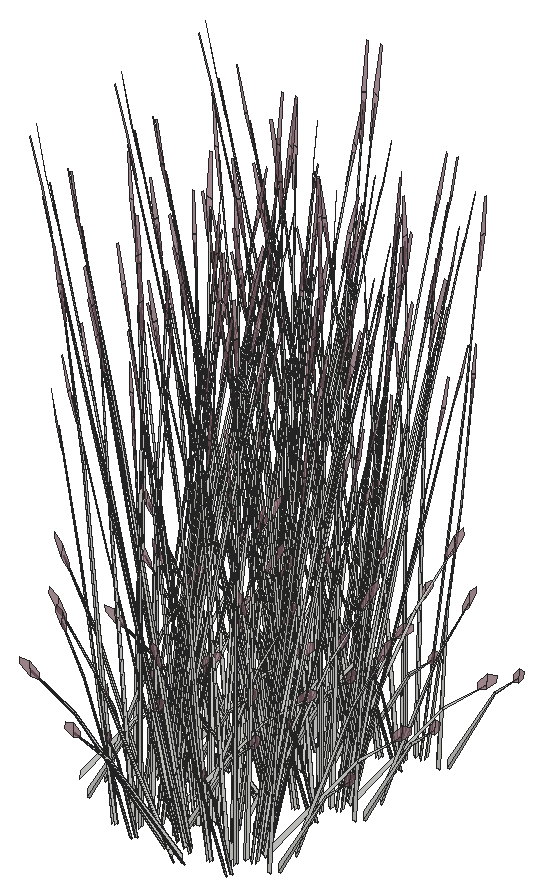
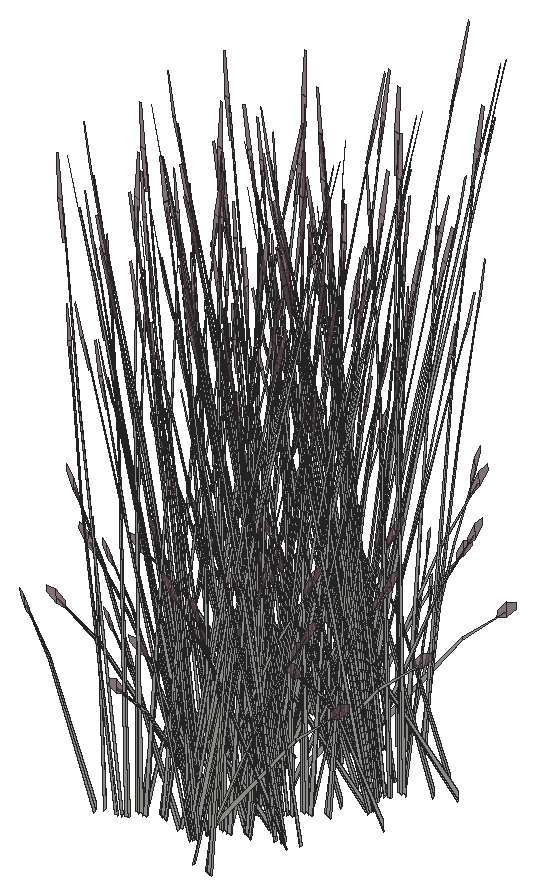
# SketchUp Ruby script. Lengths in inches.
U = 1.inch
M = Sketchup.active_model
def pt(a) = Geom::Point3d.new(a.map { |v| v * U })
def face(e, loops, mat)
  f = e.add_face(loops[0].map { |a| pt(a) })
  loops[1..].each { |l| e.add_face(l.map { |a| pt(a) }).erase! }
  f.material = f.back_material = mat if mat
  f
end
# faces: each face lists its corners as indices into pts; further lists are holes
def faces(e, pts, list, mat = nil) = list.each { |f| face(e, (f[0].is_a?(Array) ? f : [f]).map { |l| l.map { |i| pts[i] } }, mat) }
# xy, xz, yz: faces in a plane at the given z, y or x. An outline is a flat list of corners, or four numbers for a rectangle; further outlines are holes
def ring(l) = l.size == 4 ? [[l[0], l[1]], [l[2], l[1]], [l[2], l[3]], [l[0], l[3]]] : l.each_slice(2).to_a
def flat(e, list, mat, &to3) = list.each { |f| face(e, (f[0].is_a?(Array) ? f : [f]).map { |l| ring(l).map { |u, v| to3.(u, v) } }, mat) }
def xy(e, z, list, mat = nil) = flat(e, list, mat) { |x, y| [x, y, z] }
def xz(e, y, list, mat = nil) = flat(e, list, mat) { |x, z| [x, y, z] }
def yz(e, x, list, mat = nil) = flat(e, list, mat) { |y, z| [x, y, z] }
def lines(e, pts, list) = list.each { |a, b| e.add_line(pt(pts[a]), pt(pts[b])) }
# prism: a flat outline (further loops are holes) pulled along v
def prism(e, loops, v, mat = nil)
  f = face(e, loops, mat); d = Geom::Vector3d.new(v.map { |x| x * U })
  f.pushpull(f.normal.samedirection?(d) ? d.length : -d.length)
end
def box(e, o, s, mat = nil) = prism(e, [[o, [o[0] + s[0], o[1], o[2]], [o[0] + s[0], o[1] + s[1], o[2]], [o[0], o[1] + s[1], o[2]]]], [0, 0, s[2]], mat)
def at(x, y, z, deg = 0) = Geom::Transformation.translation(pt([x, y, z])) * Geom::Transformation.rotation(ORIGIN, Z_AXIS, deg.degrees)
def axes(o, x, y, z) = Geom::Transformation.new([*x, 0, *y, 0, *z, 0, *pt(o).to_a, 1])
def part(name) = M.definitions.add(name)
# library, detail: a bought-in or finely detailed component or shape, given as its bounding box
def library(name, o, s) = part(name).tap { |d| box(d.entities, o, s) }
def detail(e, o, s) = box(e.add_group.entities, o, s)
def put(e, d, t, mat = nil) = e.add_instance(d, t).tap { |i| i.material = mat if mat }
def group(e, t, mat = nil) = e.add_group.tap { |g| g.transformation = t; g.material = mat if mat }.entities
root = M.entities
M.materials.add("LightPink_Translucent").color = [144, 107, 117]
M.materials["LightPink_Translucent"].alpha = 0.75
c1 = part("blade")
p = [[2.15,0.21,22],[0,0.17,0],[0.09,0.45,0],[2.18,0.31,22],[2.29,0.31,22],[0.38,0.45,0],
  [2.48,0.24,33],[2.49,0.24,33],[2.48,0.22,33]]
faces(c1.entities,p,[[0,1,2,3],[4,5,2,3],[6,3,4,7],[8,0,3,6]])
c2 = part("seeds")
p = [[0.3,-0.1,1.38],[-0.01,-0.03,1.59],[-0.01,-0.03,0.03],[0.14,-0.07,-0.07],[0.29,-0.03,3],[0.15,0.01,3.11]]
faces(c2.entities,p,[[0,1,2,3],[1,0,4,5]],"LightPink_Translucent")
c3 = part("blade with seeds")
put(c3.entities,c1,at(0,0,0))
put(c3.entities,c2,axes([2.4,0.25,30.99],[1.5799,-0.05474,1.17369],[-0.12525,1.92788,0.29478],[-0.07173,-0.02425,1.56792]))
put(root,c3,axes([337.47,15.14,52.16],[0.03743,0.039,1.56736],[-0.18045,0.35054,-0.1481],[-0.18276,0.00254,0.27737]))
put(root,c3,axes([337.47,21.41,52.16],[0.03743,0.039,1.56736],[-0.18045,0.35054,-0.1481],[-0.18276,0.00254,0.27737]))
put(root,c3,axes([337.47,27.61,52.16],[0.03743,0.039,1.56736],[-0.18045,0.35054,-0.1481],[-0.18276,0.00254,0.27737]))
put(root,c3,axes([334.35,22.6,52.18],[0.37205,-0.1328,0.05682],[0.18211,0.24217,0.44729],[-0.03593,-0.10675,0.68204]))
put(root,c3,axes([337.88,14.91,52.17],[-0.10864,-0.00276,1.54581],[-0.34587,0.27582,-0.24447],[-0.18454,-0.05636,0.12397]))
put(root,c3,axes([337.88,21.18,52.17],[-0.10864,-0.00276,1.54581],[-0.34587,0.27582,-0.24447],[-0.18454,-0.05636,0.12397]))
put(root,c3,axes([337.88,27.37,52.17],[-0.10864,-0.00276,1.54581],[-0.34587,0.27582,-0.24447],[-0.18454,-0.05636,0.12397]))
put(root,c3,axes([330.63,17.62,52.17],[0.10831,-0.00661,1.54581],[0.29709,-0.30358,-0.24447],[0.19266,0.04007,0.12397]))
put(root,c3,axes([334.22,22.63,52.18],[0.49753,0.10215,0.42415],[-0.17013,0.33585,0.34973],[-0.0299,-0.13207,0.87768]))
put(root,c3,axes([331.58,21.97,52.16],[0.00149,-0.04731,1.56736],[0.4327,-0.20872,-0.1481],[0.1503,0.0745,0.27737]))
put(root,c3,axes([337.4375,16.43,52.18],[0.14265,-0.35629,0.42415],[0.46898,0.12183,0.34973],[-0.18443,0.02141,0.87768]))
put(root,c3,axes([337.4375,22.71,52.18],[0.14265,-0.35629,0.42415],[0.46898,0.12183,0.34973],[-0.18443,0.02141,0.87768]))
put(root,c3,axes([333.02,18.83,52.18],[0.41493,0.01821,0.05682],[-0.01138,0.27493,0.44729],[0.04342,-0.10531,0.68204]))
put(root,c3,axes([333.4,25.77,52.46],[0.15222,-0.30049,0.31292],[0.44409,0.08764,-0.40398],[0.04072,0.12098,0.77298]))
put(root,c3,axes([333.43,18.38,52.17],[-0.00487,-0.07777,1.54581],[-0.41166,-0.22476,-0.24447],[0.06364,-0.13625,0.12397]))
put(root,c3,axes([337.4,16.34,52.18],[-0.18545,-0.26643,0.05682],[0.33817,-0.13041,0.44729],[-0.14907,0.02573,0.68204]))
put(root,c3,axes([337.4,22.61,52.18],[-0.18545,-0.26643,0.05682],[0.33817,-0.13041,0.44729],[-0.14907,0.02573,0.68204]))
put(root,c3,axes([332.89,18.8,52.18],[0.35954,0.26661,0.42415],[-0.38183,0.22994,0.34973],[0.06632,-0.12508,0.87768]))
put(root,c3,axes([334.75,15,52.18],[0.37205,-0.1328,0.05682],[0.18211,0.24217,0.44729],[-0.03593,-0.10675,0.68204]))
put(root,c3,axes([333.54,19.03,52.17],[0.064,0.06292,1.54581],[0.51651,0.02472,-0.24447],[0.05194,0.13877,0.12397]))
put(root,c3,axes([334.62,15.03,52.18],[0.49753,0.10215,0.42415],[-0.17013,0.33585,0.34973],[-0.0299,-0.13207,0.87768]))
put(root,c3,axes([337.55,17.32,52.18],[-0.12522,-0.35963,0.42415],[0.49122,-0.06241,0.34973],[-0.14477,0.08458,0.87768]))
put(root,c3,axes([337.55,23.59,52.18],[-0.12522,-0.35963,0.42415],[0.49122,-0.06241,0.34973],[-0.14477,0.08458,0.87768]))
put(root,c3,axes([333.81,18.18,52.46],[0.15222,-0.30049,0.31292],[0.44409,0.08764,-0.40398],[0.04072,0.12098,0.77298]))
put(root,c3,axes([333.3,19.65,52.46],[-0.43951,0.05584,0.31292],[-0.11606,-0.31924,-0.40398],[0.12595,-0.08575,0.77298]))
put(root,c3,axes([337.8,15.53,52.5],[0.41698,-0.28837,0.47505],[0.35962,0.30624,0.3917],[-0.19563,-0.05319,0.983]))
put(root,c3,axes([337.8,21.8,52.5],[0.41698,-0.28837,0.47505],[0.35962,0.30624,0.3917],[-0.19563,-0.05319,0.983]))
put(root,c3,axes([337.8,28,52.5],[0.41698,-0.28837,0.47505],[0.35962,0.30624,0.3917],[-0.19563,-0.05319,0.983]))
put(root,c3,axes([331.76,18.17,52.16],[-0.04566,-0.03421,1.56736],[0.09987,-0.36669,-0.1481],[0.17984,-0.02343,0.27737]))
put(root,c3,axes([334,26.85,52.99],[0.34892,-0.22417,-0.05733],[0.3197,0.24551,-0.25992],[0.02251,0.06957,0.85731]))
put(root,c3,axes([337.45,17.25,52.18],[-0.34663,-0.16434,0.05682],[0.20181,-0.23402,0.44729],[-0.11113,0.07566,0.68204]))
put(root,c3,axes([337.45,23.52,52.18],[-0.34663,-0.16434,0.05682],[0.20181,-0.23402,0.44729],[-0.11113,0.07566,0.68204]))
put(root,c3,axes([336.05,26.65,52.46],[-0.15222,0.30049,0.31292],[-0.44409,-0.08764,-0.40398],[-0.04072,-0.12098,0.77298]))
put(root,c3,axes([335.28,30.35,52.18],[0.37205,-0.1328,0.05682],[0.18211,0.24217,0.44729],[-0.03593,-0.10675,0.68204]))
put(root,c3,axes([335.78,22.3,52.16],[-0.05128,0.02985,1.56736],[-0.5024,-0.1007,-0.1481],[-0.01819,-0.13025,0.27737]))
put(root,c3,axes([335.15,30.37,52.18],[0.49753,0.10215,0.42415],[-0.17013,0.33585,0.34973],[-0.0299,-0.13207,0.87768]))
put(root,c3,axes([337.78,16.4375,52.46],[0.41962,0.10901,0.31292],[-0.12239,0.31802,-0.40398],[-0.16894,0.02916,0.77298]))
put(root,c3,axes([337.78,22.71,52.46],[0.41962,0.10901,0.31292],[-0.12239,0.31802,-0.40398],[-0.16894,0.02916,0.77298]))
put(root,c3,axes([334.4,19.25,52.99],[0.34892,-0.22417,-0.05733],[0.3197,0.24551,-0.25992],[0.02251,0.06957,0.85731]))
put(root,c3,axes([332.13,16.57,52.17],[0.07006,-0.05952,1.54581],[-0.08968,-0.3651,-0.24447],[0.1758,-0.06922,0.12397]))
put(root,c3,axes([337.99,15.53,52.18],[0.02542,-0.29714,0.05682],[0.38391,0.00815,0.44729],[-0.14706,-0.03109,0.68204]))
put(root,c3,axes([337.99,21.8,52.18],[0.02542,-0.29714,0.05682],[0.38391,0.00815,0.44729],[-0.14706,-0.03109,0.68204]))
put(root,c3,axes([337.99,27.99,52.18],[0.02542,-0.29714,0.05682],[0.38391,0.00815,0.44729],[-0.14706,-0.03109,0.68204]))
put(root,c3,axes([337.09,18.07,52.17],[-0.01255,0.07733,1.54581],[0.35618,0.269,-0.24447],[-0.09325,0.12721,0.12397]))
put(root,c3,axes([337.09,24.34,52.17],[-0.01255,0.07733,1.54581],[0.35618,0.269,-0.24447],[-0.09325,0.12721,0.12397]))
put(root,c3,axes([335.17,23.21,52.46],[-0.34164,0.20573,0.31292],[-0.3234,-0.23491,-0.40398],[0.04921,-0.11936,0.77298]))
put(root,c3,axes([339.18,15.02,52.8],[-0.33698,0.3746,-0.12034],[-0.48801,-0.21581,-0.66795],[-0.16964,-0.10584,1.01494]))
put(root,c3,axes([339.18,21.29,52.8],[-0.33698,0.3746,-0.12034],[-0.48801,-0.21581,-0.66795],[-0.16964,-0.10584,1.01494]))
put(root,c3,axes([339.18,27.48,52.8],[-0.33698,0.3746,-0.12034],[-0.48801,-0.21581,-0.66795],[-0.16964,-0.10584,1.01494]))
put(root,c3,axes([332.9,21.1,52.46],[-0.28729,-0.24465,0.31292],[0.32804,-0.23159,-0.40398],[0.16667,0.03524,0.77298]))
put(root,c3,axes([338.25,15.75,52.46],[0.28729,0.24465,0.31292],[-0.32804,0.23159,-0.40398],[-0.16667,-0.03524,0.77298]))
put(root,c3,axes([338.25,22.02,52.46],[0.28729,0.24465,0.31292],[-0.32804,0.23159,-0.40398],[-0.16667,-0.03524,0.77298]))
put(root,c3,axes([338.25,28.22,52.46],[0.28729,0.24465,0.31292],[-0.32804,0.23159,-0.40398],[-0.16667,-0.03524,0.77298]))
put(root,c3,axes([336.18,14.7,52.16],[-0.05128,0.02985,1.56736],[-0.5024,-0.1007,-0.1481],[-0.01819,-0.13025,0.27737]))
put(root,c3,axes([333.16,21.32,52.18],[-0.02542,0.29714,0.05682],[-0.38391,-0.00815,0.44729],[0.14706,0.03109,0.68204]))
put(root,c3,axes([333.2,21.23,52.18],[-0.3723,0.25748,0.42415],[-0.32109,-0.27343,0.34973],[0.17467,0.04749,0.87768]))
put(root,c3,axes([333.375,20.42,52.46],[-0.41962,-0.10901,0.31292],[0.12239,-0.31802,-0.40398],[0.16894,-0.02916,0.77298]))
put(root,c3,axes([335.57,15.62,52.46],[-0.34164,0.20573,0.31292],[-0.3234,-0.23491,-0.40398],[0.04921,-0.11936,0.77298]))
put(root,c3,axes([334.64,25.94,52.18],[-0.5022,0.08967,0.42415],[-0.08716,-0.35177,0.34973],[0.11811,0.10367,0.87768]))
put(root,c3,axes([334.54,26.01,52.18],[-0.22948,0.24822,0.05682],[-0.32679,-0.14452,0.44729],[0.10565,0.07958,0.68204]))
put(root,c3,axes([336.19,26.375,52.18],[0.37205,-0.1328,0.05682],[0.18211,0.24217,0.44729],[-0.03593,-0.10675,0.68204]))
put(root,c3,axes([336.85,18.11,52.99],[0.44556,0.1043,-0.05733],[-0.13706,0.32103,-0.25992],[-0.07288,0.04874,0.85731]))
put(root,c3,axes([336.85,24.38,52.99],[0.44556,0.1043,-0.05733],[-0.13706,0.32103,-0.25992],[-0.07288,0.04874,0.85731]))
put(root,c3,axes([333.7,19.6,52.18],[0.34663,0.16434,0.05682],[-0.20181,0.23402,0.44729],[0.11113,-0.07566,0.68204]))
put(root,c3,axes([336.06,26.4,52.18],[0.49753,0.10215,0.42415],[-0.17013,0.33585,0.34973],[-0.0299,-0.13207,0.87768]))
put(root,c3,axes([336.71,30.04,52.16],[-0.05128,0.02985,1.56736],[-0.5024,-0.1007,-0.1481],[-0.01819,-0.13025,0.27737]))
put(root,c3,axes([337.85,17.2,52.46],[0.43951,-0.05584,0.31292],[0.11606,0.31924,-0.40398],[-0.12595,0.08575,0.77298]))
put(root,c3,axes([337.85,23.47,52.46],[0.43951,-0.05584,0.31292],[0.11606,0.31924,-0.40398],[-0.12595,0.08575,0.77298]))
put(root,c3,axes([333.61,19.53,52.18],[0.12522,0.35963,0.42415],[-0.49122,0.06241,0.34973],[0.14477,-0.08458,0.87768]))
put(root,c3,axes([335.04,18.34,52.18],[-0.5022,0.08967,0.42415],[-0.08716,-0.35177,0.34973],[0.11811,0.10367,0.87768]))
put(root,c3,axes([334.94,18.41,52.18],[-0.22948,0.24822,0.05682],[-0.32679,-0.14452,0.44729],[0.10565,0.07958,0.68204]))
put(root,c3,axes([339.05,14.125,52.16],[-0.00942,0.04684,1.56736],[-0.46458,0.16998,-0.1481],[-0.13671,-0.08689,0.27737]))
put(root,c3,axes([339.05,20.4,52.16],[-0.00942,0.04684,1.56736],[-0.46458,0.16998,-0.1481],[-0.13671,-0.08689,0.27737]))
put(root,c3,axes([339.05,26.59,52.16],[-0.00942,0.04684,1.56736],[-0.46458,0.16998,-0.1481],[-0.13671,-0.08689,0.27737]))
put(root,c3,axes([334.68,19.59,52.16],[-0.06595,-0.00297,1.56736],[-0.27386,-0.31799,-0.1481],[0.10998,-0.10455,0.27737]))
put(root,c3,axes([334.47,25.72,52.46],[-0.07798,-0.31474,0.31292],[0.44579,-0.08311,-0.40398],[0.11974,0.09019,0.77298]))
put(root,c3,axes([338.27,18.05,52.18],[-0.35954,-0.26661,0.42415],[0.38183,-0.22994,0.34973],[-0.06632,0.12508,0.87768]))
put(root,c3,axes([338.27,24.32,52.18],[-0.35954,-0.26661,0.42415],[0.38183,-0.22994,0.34973],[-0.06632,0.12508,0.87768]))
put(root,c3,axes([333.75,20.51,52.18],[0.18545,0.26643,0.05682],[-0.33817,0.13041,0.44729],[0.14907,-0.02573,0.68204]))
put(root,c3,axes([338.14,18.02,52.18],[-0.41493,-0.01821,0.05682],[0.01138,-0.27493,0.44729],[-0.04342,0.10531,0.68204]))
put(root,c3,axes([338.14,24.3,52.18],[-0.41493,-0.01821,0.05682],[0.01138,-0.27493,0.44729],[-0.04342,0.10531,0.68204]))
put(root,c3,axes([333.72,20.42,52.18],[-0.14265,0.35629,0.42415],[-0.46898,-0.12183,0.34973],[0.18443,-0.02141,0.87768]))
put(root,c3,axes([334.04,26.16,52.16],[0.00149,-0.04731,1.56736],[0.4327,-0.20872,-0.1481],[0.1503,0.0745,0.27737]))
put(root,c3,axes([335.48,23.03,52.18],[0.41493,0.01821,0.05682],[-0.01138,0.27493,0.44729],[0.04342,-0.10531,0.68204]))
put(root,c3,axes([335.89,22.57,52.17],[-0.00487,-0.07777,1.54581],[-0.41166,-0.22476,-0.24447],[0.06364,-0.13625,0.12397]))
put(root,c3,axes([335.34,23,52.18],[0.35954,0.26661,0.42415],[-0.38183,0.22994,0.34973],[0.06632,-0.12508,0.87768]))
put(root,c3,axes([339.14,15.33,52.46],[0.07798,0.31474,0.31292],[-0.44579,0.08311,-0.40398],[-0.11974,-0.09019,0.77298]))
put(root,c3,axes([339.14,21.6,52.46],[0.07798,0.31474,0.31292],[-0.44579,0.08311,-0.40398],[-0.11974,-0.09019,0.77298]))
put(root,c3,axes([339.14,27.79,52.46],[0.07798,0.31474,0.31292],[-0.44579,0.08311,-0.40398],[-0.11974,-0.09019,0.77298]))
put(root,c3,axes([334.87,18.125,52.46],[-0.07798,-0.31474,0.31292],[0.44579,-0.08311,-0.40398],[0.11974,0.09019,0.77298]))
put(root,c3,axes([337.05,18.86,52.16],[0.05728,-0.02359,1.56736],[0.47345,0.15692,-0.1481],[-0.01113,0.13066,0.27737]))
put(root,c3,axes([337.05,25.13,52.16],[0.05728,-0.02359,1.56736],[0.47345,0.15692,-0.1481],[-0.01113,0.13066,0.27737]))
put(root,c3,axes([337.62,26.07,52.16],[-0.05128,0.02985,1.56736],[-0.5024,-0.1007,-0.1481],[-0.01819,-0.13025,0.27737]))
put(root,c3,axes([333.42,21.02,52.17],[0.10831,-0.00661,1.54581],[0.29709,-0.30358,-0.24447],[0.19266,0.04007,0.12397]))
put(root,c3,axes([334.4375,18.57,52.16],[0.00149,-0.04731,1.56736],[0.4327,-0.20872,-0.1481],[0.1503,0.0745,0.27737]))
put(root,c3,axes([335.88,15.43,52.18],[0.41493,0.01821,0.05682],[-0.01138,0.27493,0.44729],[0.04342,-0.10531,0.68204]))
put(root,c3,axes([337.01,26.99,52.46],[-0.34164,0.20573,0.31292],[-0.3234,-0.23491,-0.40398],[0.04921,-0.11936,0.77298]))
put(root,c3,axes([336.29,14.98,52.17],[-0.00487,-0.07777,1.54581],[-0.41166,-0.22476,-0.24447],[0.06364,-0.13625,0.12397]))
put(root,c3,axes([338.94,14.96,52.5],[0.56246,-0.10044,0.47505],[0.09762,0.39398,0.3917],[-0.13228,-0.11611,0.983]))
put(root,c3,axes([338.94,21.23,52.5],[0.56246,-0.10044,0.47505],[0.09762,0.39398,0.3917],[-0.13228,-0.11611,0.983]))
put(root,c3,axes([338.94,27.42,52.5],[0.56246,-0.10044,0.47505],[0.09762,0.39398,0.3917],[-0.13228,-0.11611,0.983]))
put(root,c3,axes([335.76,23.85,52.46],[-0.43951,0.05584,0.31292],[-0.11606,-0.31924,-0.40398],[0.12595,-0.08575,0.77298]))
put(root,c3,axes([335.75,15.4,52.18],[0.35954,0.26661,0.42415],[-0.38183,0.22994,0.34973],[0.06632,-0.12508,0.87768]))
put(root,c3,axes([339.07,15.04,52.18],[0.22948,-0.24822,0.05682],[0.32679,0.14452,0.44729],[-0.10565,-0.07958,0.68204]))
put(root,c3,axes([339.07,21.3125,52.18],[0.22948,-0.24822,0.05682],[0.32679,0.14452,0.44729],[-0.10565,-0.07958,0.68204]))
put(root,c3,axes([339.07,27.51,52.18],[0.22948,-0.24822,0.05682],[0.32679,0.14452,0.44729],[-0.10565,-0.07958,0.68204]))
put(root,c3,axes([334.5625,21.57,52.16],[-0.04566,-0.03421,1.56736],[0.09987,-0.36669,-0.1481],[0.17984,-0.02343,0.27737]))
put(root,c3,axes([336.16,16.25,52.46],[-0.43951,0.05584,0.31292],[-0.11606,-0.31924,-0.40398],[0.12595,-0.08575,0.77298]))
put(root,c3,axes([339.57,14.3,52.17],[-0.07723,-0.05479,1.54581],[-0.51538,0.03473,-0.24447],[-0.08225,-0.13104,0.12397]))
put(root,c3,axes([339.57,20.58,52.17],[-0.07723,-0.05479,1.54581],[-0.51538,0.03473,-0.24447],[-0.08225,-0.13104,0.12397]))
put(root,c3,axes([339.57,26.77,52.17],[-0.07723,-0.05479,1.54581],[-0.51538,0.03473,-0.24447],[-0.08225,-0.13104,0.12397]))
put(root,c3,axes([335.36,25.3,52.46],[-0.28729,-0.24465,0.31292],[0.32804,-0.23159,-0.40398],[0.16667,0.03524,0.77298]))
put(root,c3,axes([338.45,17.84,52.46],[0.34164,-0.20573,0.31292],[0.3234,0.23491,-0.40398],[-0.04921,0.11936,0.77298]))
put(root,c3,axes([338.45,24.11,52.46],[0.34164,-0.20573,0.31292],[0.3234,0.23491,-0.40398],[-0.04921,0.11936,0.77298]))
put(root,c3,axes([335.62,25.52,52.18],[-0.02542,0.29714,0.05682],[-0.38391,-0.00815,0.44729],[0.14706,0.03109,0.68204]))
put(root,c3,axes([334.93,19.97,52.17],[0.07006,-0.05952,1.54581],[-0.08968,-0.3651,-0.24447],[0.1758,-0.06922,0.12397]))
put(root,c3,axes([335.65,25.43,52.18],[-0.3723,0.25748,0.42415],[-0.32109,-0.27343,0.34973],[0.17467,0.04749,0.87768]))
put(root,c3,axes([335.83,24.61,52.46],[-0.41962,-0.10901,0.31292],[0.12239,-0.31802,-0.40398],[0.16894,-0.02916,0.77298]))
put(root,c3,axes([338.23,17.89,52.77],[0.55492,0.01936,-0.11927],[-0.01517,0.36657,-0.66198],[-0.03855,0.14118,1.00587]))
put(root,c3,axes([338.23,24.17,52.77],[0.55492,0.01936,-0.11927],[-0.01517,0.36657,-0.66198],[-0.03855,0.14118,1.00587]))
put(root,c3,axes([335.76,17.7,52.46],[-0.28729,-0.24465,0.31292],[0.32804,-0.23159,-0.40398],[0.16667,0.03524,0.77298]))
put(root,c3,axes([336.02,17.92,52.18],[-0.02542,0.29714,0.05682],[-0.38391,-0.00815,0.44729],[0.14706,0.03109,0.68204]))
put(root,c3,axes([336.06,17.83,52.18],[-0.3723,0.25748,0.42415],[-0.32109,-0.27343,0.34973],[0.17467,0.04749,0.87768]))
put(root,c3,axes([336.16,23.8,52.18],[0.34663,0.16434,0.05682],[-0.20181,0.23402,0.44729],[0.11113,-0.07566,0.68204]))
put(root,c3,axes([337.32,26.8,52.18],[0.41493,0.01821,0.05682],[-0.01138,0.27493,0.44729],[0.04342,-0.10531,0.68204]))
put(root,c3,axes([336.23,17.01,52.46],[-0.41962,-0.10901,0.31292],[0.12239,-0.31802,-0.40398],[0.16894,-0.02916,0.77298]))
put(root,c3,axes([336.0625,23.73,52.18],[0.12522,0.35963,0.42415],[-0.49122,0.06241,0.34973],[0.14477,-0.08458,0.87768]))
put(root,c3,axes([337.73,26.35,52.17],[-0.00487,-0.07777,1.54581],[-0.41166,-0.22476,-0.24447],[0.06364,-0.13625,0.12397]))
put(root,c3,axes([337.1875,26.77,52.18],[0.35954,0.26661,0.42415],[-0.38183,0.22994,0.34973],[0.06632,-0.12508,0.87768]))
put(root,c3,axes([337.14,23.79,52.16],[-0.06595,-0.00297,1.56736],[-0.27386,-0.31799,-0.1481],[0.10998,-0.10455,0.27737]))
put(root,c3,axes([336.5625,16.2,52.18],[0.34663,0.16434,0.05682],[-0.20181,0.23402,0.44729],[0.11113,-0.07566,0.68204]))
put(root,c3,axes([336.21,24.71,52.18],[0.18545,0.26643,0.05682],[-0.33817,0.13041,0.44729],[0.14907,-0.02573,0.68204]))
put(root,c3,axes([340.21,15.28,52.46],[-0.15222,0.30049,0.31292],[-0.44409,-0.08764,-0.40398],[-0.04072,-0.12098,0.77298]))
put(root,c3,axes([340.21,21.55,52.46],[-0.15222,0.30049,0.31292],[-0.44409,-0.08764,-0.40398],[-0.04072,-0.12098,0.77298]))
put(root,c3,axes([340.21,27.74,52.46],[-0.15222,0.30049,0.31292],[-0.44409,-0.08764,-0.40398],[-0.04072,-0.12098,0.77298]))
put(root,c3,axes([336.47,16.13,52.18],[0.12522,0.35963,0.42415],[-0.49122,0.06241,0.34973],[0.14477,-0.08458,0.87768]))
put(root,c3,axes([336.18,24.62,52.18],[-0.14265,0.35629,0.42415],[-0.46898,-0.12183,0.34973],[0.18443,-0.02141,0.87768]))
put(root,c3,axes([337.6,27.62,52.46],[-0.43951,0.05584,0.31292],[-0.11606,-0.31924,-0.40398],[0.12595,-0.08575,0.77298]))
put(root,c3,axes([339.4,18.42,52.47],[-0.49753,-0.10215,0.47081],[0.17013,-0.33585,0.3882],[0.0299,0.13207,0.97422]))
put(root,c3,axes([339.4,24.69,52.47],[-0.49753,-0.10215,0.47081],[0.17013,-0.33585,0.3882],[0.0299,0.13207,0.97422]))
put(root,c3,axes([339.27,18.45,52.18],[-0.37205,0.1328,0.05682],[-0.18211,-0.24217,0.44729],[0.03593,0.10675,0.68204]))
put(root,c3,axes([339.27,24.72,52.18],[-0.37205,0.1328,0.05682],[-0.18211,-0.24217,0.44729],[0.03593,0.10675,0.68204]))
put(root,c3,axes([337.54,16.1875,52.16],[-0.06595,-0.00297,1.56736],[-0.27386,-0.31799,-0.1481],[0.10998,-0.10455,0.27737]))
put(root,c3,axes([336.61,17.11,52.18],[0.18545,0.26643,0.05682],[-0.33817,0.13041,0.44729],[0.14907,-0.02573,0.68204]))
put(root,c3,axes([335.88,25.22,52.17],[0.10831,-0.00661,1.54581],[0.29709,-0.30358,-0.24447],[0.19266,0.04007,0.12397]))
put(root,c3,axes([336.58,17.02,52.18],[-0.14265,0.35629,0.42415],[-0.46898,-0.12183,0.34973],[0.18443,-0.02141,0.87768]))
put(root,c3,axes([336.28,17.62,52.17],[0.10831,-0.00661,1.54581],[0.29709,-0.30358,-0.24447],[0.19266,0.04007,0.12397]))
put(root,c3,axes([337.67,28.38,52.46],[-0.41962,-0.10901,0.31292],[0.12239,-0.31802,-0.40398],[0.16894,-0.02916,0.77298]))
put(root,c3,axes([337.02,25.77,52.16],[-0.04566,-0.03421,1.56736],[0.09987,-0.36669,-0.1481],[0.17984,-0.02343,0.27737]))
put(root,c3,axes([340.35,15,52.18],[0.37205,-0.1328,0.05682],[0.18211,0.24217,0.44729],[-0.03593,-0.10675,0.68204]))
put(root,c3,axes([340.35,21.28,52.18],[0.37205,-0.1328,0.05682],[0.18211,0.24217,0.44729],[-0.03593,-0.10675,0.68204]))
put(root,c3,axes([340.35,27.47,52.18],[0.37205,-0.1328,0.05682],[0.18211,0.24217,0.44729],[-0.03593,-0.10675,0.68204]))
put(root,c3,axes([339.14,19.03,52.17],[0.064,0.06292,1.54581],[0.51651,0.02472,-0.24447],[0.05194,0.13877,0.12397]))
put(root,c3,axes([339.14,25.3,52.17],[0.064,0.06292,1.54581],[0.51651,0.02472,-0.24447],[0.05194,0.13877,0.12397]))
put(root,c3,axes([340.22,15.03,52.18],[0.49753,0.10215,0.42415],[-0.17013,0.33585,0.34973],[-0.0299,-0.13207,0.87768]))
put(root,c3,axes([340.22,21.3,52.18],[0.49753,0.10215,0.42415],[-0.17013,0.33585,0.34973],[-0.0299,-0.13207,0.87768]))
put(root,c3,axes([340.22,27.49,52.18],[0.49753,0.10215,0.42415],[-0.17013,0.33585,0.34973],[-0.0299,-0.13207,0.87768]))
put(root,c3,axes([339.4,18.18,52.46],[0.15222,-0.30049,0.31292],[0.44409,0.08764,-0.40398],[0.04072,0.12098,0.77298]))
put(root,c3,axes([339.4,24.45,52.46],[0.15222,-0.30049,0.31292],[0.44409,0.08764,-0.40398],[0.04072,0.12098,0.77298]))
put(root,c3,axes([338,27.57,52.18],[0.34663,0.16434,0.05682],[-0.20181,0.23402,0.44729],[0.11113,-0.07566,0.68204]))
put(root,c3,axes([337.91,27.5,52.18],[0.12522,0.35963,0.42415],[-0.49122,0.06241,0.34973],[0.14477,-0.08458,0.87768]))
put(root,c3,axes([337.42,18.17,52.16],[-0.04566,-0.03421,1.56736],[0.09987,-0.36669,-0.1481],[0.17984,-0.02343,0.27737]))
put(root,c3,axes([337.39,24.17,52.17],[0.07006,-0.05952,1.54581],[-0.08968,-0.3651,-0.24447],[0.1758,-0.06922,0.12397]))
put(root,c3,axes([338.98,27.56,52.16],[-0.06595,-0.00297,1.56736],[-0.27386,-0.31799,-0.1481],[0.10998,-0.10455,0.27737]))
put(root,c3,axes([338.05,28.48,52.18],[0.18545,0.26643,0.05682],[-0.33817,0.13041,0.44729],[0.14907,-0.02573,0.68204]))
put(root,c3,axes([340,19.25,52.99],[0.34892,-0.22417,-0.05733],[0.3197,0.24551,-0.25992],[0.02251,0.06957,0.85731]))
put(root,c3,axes([340,25.52,52.99],[0.34892,-0.22417,-0.05733],[0.3197,0.24551,-0.25992],[0.02251,0.06957,0.85731]))
put(root,c3,axes([338.02,28.39,52.18],[-0.14265,0.35629,0.42415],[-0.46898,-0.12183,0.34973],[0.18443,-0.02141,0.87768]))
put(root,c3,axes([337.79,16.57,52.17],[0.07006,-0.05952,1.54581],[-0.08968,-0.3651,-0.24447],[0.1758,-0.06922,0.12397]))
put(root,c3,axes([341.78,14.7,52.16],[-0.05128,0.02985,1.56736],[-0.5024,-0.1007,-0.1481],[-0.01819,-0.13025,0.27737]))
put(root,c3,axes([341.78,20.97,52.16],[-0.05128,0.02985,1.56736],[-0.5024,-0.1007,-0.1481],[-0.01819,-0.13025,0.27737]))
put(root,c3,axes([341.78,27.16,52.16],[-0.05128,0.02985,1.56736],[-0.5024,-0.1007,-0.1481],[-0.01819,-0.13025,0.27737]))
put(root,c3,axes([341.17,15.62,52.46],[-0.34164,0.20573,0.31292],[-0.3234,-0.23491,-0.40398],[0.04921,-0.11936,0.77298]))
put(root,c3,axes([341.17,21.89,52.46],[-0.34164,0.20573,0.31292],[-0.3234,-0.23491,-0.40398],[0.04921,-0.11936,0.77298]))
put(root,c3,axes([341.17,28.08,52.46],[-0.34164,0.20573,0.31292],[-0.3234,-0.23491,-0.40398],[0.04921,-0.11936,0.77298]))
put(root,c3,axes([340.64,18.34,52.18],[-0.5022,0.08967,0.42415],[-0.08716,-0.35177,0.34973],[0.11811,0.10367,0.87768]))
put(root,c3,axes([340.64,24.61,52.18],[-0.5022,0.08967,0.42415],[-0.08716,-0.35177,0.34973],[0.11811,0.10367,0.87768]))
put(root,c3,axes([340.54,18.41,52.18],[-0.22948,0.24822,0.05682],[-0.32679,-0.14452,0.44729],[0.10565,0.07958,0.68204]))
put(root,c3,axes([340.54,24.68,52.18],[-0.22948,0.24822,0.05682],[-0.32679,-0.14452,0.44729],[0.10565,0.07958,0.68204]))
put(root,c3,axes([339.23,27.9375,52.17],[0.07006,-0.05952,1.54581],[-0.08968,-0.3651,-0.24447],[0.1758,-0.06922,0.12397]))
put(root,c3,axes([340.47,18.125,52.46],[-0.07798,-0.31474,0.31292],[0.44579,-0.08311,-0.40398],[0.11974,0.09019,0.77298]))
put(root,c3,axes([340.47,24.4,52.46],[-0.07798,-0.31474,0.31292],[0.44579,-0.08311,-0.40398],[0.11974,0.09019,0.77298]))
put(root,c3,axes([340.04,18.57,52.16],[0.00149,-0.04731,1.56736],[0.4327,-0.20872,-0.1481],[0.1503,0.0745,0.27737]))
put(root,c3,axes([340.04,24.84,52.16],[0.00149,-0.04731,1.56736],[0.4327,-0.20872,-0.1481],[0.1503,0.0745,0.27737]))
put(root,c3,axes([341.48,15.43,52.18],[0.41493,0.01821,0.05682],[-0.01138,0.27493,0.44729],[0.04342,-0.10531,0.68204]))
put(root,c3,axes([341.48,21.7,52.18],[0.41493,0.01821,0.05682],[-0.01138,0.27493,0.44729],[0.04342,-0.10531,0.68204]))
put(root,c3,axes([341.48,27.89,52.18],[0.41493,0.01821,0.05682],[-0.01138,0.27493,0.44729],[0.04342,-0.10531,0.68204]))
put(root,c3,axes([341.89,14.98,52.17],[-0.00487,-0.07777,1.54581],[-0.41166,-0.22476,-0.24447],[0.06364,-0.13625,0.12397]))
put(root,c3,axes([341.89,21.25,52.17],[-0.00487,-0.07777,1.54581],[-0.41166,-0.22476,-0.24447],[0.06364,-0.13625,0.12397]))
put(root,c3,axes([341.89,27.44,52.17],[-0.00487,-0.07777,1.54581],[-0.41166,-0.22476,-0.24447],[0.06364,-0.13625,0.12397]))
put(root,c3,axes([341.34,15.4,52.18],[0.35954,0.26661,0.42415],[-0.38183,0.22994,0.34973],[0.06632,-0.12508,0.87768]))
put(root,c3,axes([341.34,21.68,52.18],[0.35954,0.26661,0.42415],[-0.38183,0.22994,0.34973],[0.06632,-0.12508,0.87768]))
put(root,c3,axes([341.34,27.87,52.18],[0.35954,0.26661,0.42415],[-0.38183,0.22994,0.34973],[0.06632,-0.12508,0.87768]))
put(root,c3,axes([341.76,16.25,52.46],[-0.43951,0.05584,0.31292],[-0.11606,-0.31924,-0.40398],[0.12595,-0.08575,0.77298]))
put(root,c3,axes([341.76,22.52,52.46],[-0.43951,0.05584,0.31292],[-0.11606,-0.31924,-0.40398],[0.12595,-0.08575,0.77298]))
put(root,c3,axes([341.76,28.72,52.46],[-0.43951,0.05584,0.31292],[-0.11606,-0.31924,-0.40398],[0.12595,-0.08575,0.77298]))
put(root,c3,axes([341.36,17.7,52.46],[-0.28729,-0.24465,0.31292],[0.32804,-0.23159,-0.40398],[0.16667,0.03524,0.77298]))
put(root,c3,axes([341.36,23.97,52.46],[-0.28729,-0.24465,0.31292],[0.32804,-0.23159,-0.40398],[0.16667,0.03524,0.77298]))
put(root,c3,axes([341.62,17.92,52.18],[-0.02542,0.29714,0.05682],[-0.38391,-0.00815,0.44729],[0.14706,0.03109,0.68204]))
put(root,c3,axes([341.62,24.19,52.18],[-0.02542,0.29714,0.05682],[-0.38391,-0.00815,0.44729],[0.14706,0.03109,0.68204]))
put(root,c3,axes([341.65,17.83,52.18],[-0.3723,0.25748,0.42415],[-0.32109,-0.27343,0.34973],[0.17467,0.04749,0.87768]))
put(root,c3,axes([341.65,24.1,52.18],[-0.3723,0.25748,0.42415],[-0.32109,-0.27343,0.34973],[0.17467,0.04749,0.87768]))
put(root,c3,axes([341.83,17.01,52.46],[-0.41962,-0.10901,0.31292],[0.12239,-0.31802,-0.40398],[0.16894,-0.02916,0.77298]))
put(root,c3,axes([341.83,23.29,52.46],[-0.41962,-0.10901,0.31292],[0.12239,-0.31802,-0.40398],[0.16894,-0.02916,0.77298]))
put(root,c3,axes([342.16,16.2,52.18],[0.34663,0.16434,0.05682],[-0.20181,0.23402,0.44729],[0.11113,-0.07566,0.68204]))
put(root,c3,axes([342.16,22.47,52.18],[0.34663,0.16434,0.05682],[-0.20181,0.23402,0.44729],[0.11113,-0.07566,0.68204]))
put(root,c3,axes([342.16,28.67,52.18],[0.34663,0.16434,0.05682],[-0.20181,0.23402,0.44729],[0.11113,-0.07566,0.68204]))
put(root,c3,axes([342.0625,16.13,52.18],[0.12522,0.35963,0.42415],[-0.49122,0.06241,0.34973],[0.14477,-0.08458,0.87768]))
put(root,c3,axes([342.0625,22.4,52.18],[0.12522,0.35963,0.42415],[-0.49122,0.06241,0.34973],[0.14477,-0.08458,0.87768]))
put(root,c3,axes([342.0625,28.6,52.18],[0.12522,0.35963,0.42415],[-0.49122,0.06241,0.34973],[0.14477,-0.08458,0.87768]))
put(root,c3,axes([343.14,16.1875,52.16],[-0.06595,-0.00297,1.56736],[-0.27386,-0.31799,-0.1481],[0.10998,-0.10455,0.27737]))
put(root,c3,axes([343.14,22.46,52.16],[-0.06595,-0.00297,1.56736],[-0.27386,-0.31799,-0.1481],[0.10998,-0.10455,0.27737]))
put(root,c3,axes([343.14,28.65,52.16],[-0.06595,-0.00297,1.56736],[-0.27386,-0.31799,-0.1481],[0.10998,-0.10455,0.27737]))
put(root,c3,axes([342.21,17.11,52.18],[0.18545,0.26643,0.05682],[-0.33817,0.13041,0.44729],[0.14907,-0.02573,0.68204]))
put(root,c3,axes([342.21,23.39,52.18],[0.18545,0.26643,0.05682],[-0.33817,0.13041,0.44729],[0.14907,-0.02573,0.68204]))
put(root,c3,axes([342.18,17.02,52.18],[-0.14265,0.35629,0.42415],[-0.46898,-0.12183,0.34973],[0.18443,-0.02141,0.87768]))
put(root,c3,axes([342.18,23.29,52.18],[-0.14265,0.35629,0.42415],[-0.46898,-0.12183,0.34973],[0.18443,-0.02141,0.87768]))
put(root,c3,axes([341.88,17.62,52.17],[0.10831,-0.00661,1.54581],[0.29709,-0.30358,-0.24447],[0.19266,0.04007,0.12397]))
put(root,c3,axes([341.88,23.89,52.17],[0.10831,-0.00661,1.54581],[0.29709,-0.30358,-0.24447],[0.19266,0.04007,0.12397]))
put(root,c3,axes([343.02,18.17,52.16],[-0.04566,-0.03421,1.56736],[0.09987,-0.36669,-0.1481],[0.17984,-0.02343,0.27737]))
put(root,c3,axes([343.02,24.44,52.16],[-0.04566,-0.03421,1.56736],[0.09987,-0.36669,-0.1481],[0.17984,-0.02343,0.27737]))
put(root,c3,axes([343.39,16.57,52.17],[0.07006,-0.05952,1.54581],[-0.08968,-0.3651,-0.24447],[0.1758,-0.06922,0.12397]))
put(root,c3,axes([343.39,22.84,52.17],[0.07006,-0.05952,1.54581],[-0.08968,-0.3651,-0.24447],[0.1758,-0.06922,0.12397]))
put(root,c3,axes([343.39,29.03,52.17],[0.07006,-0.05952,1.54581],[-0.08968,-0.3651,-0.24447],[0.1758,-0.06922,0.12397]))
